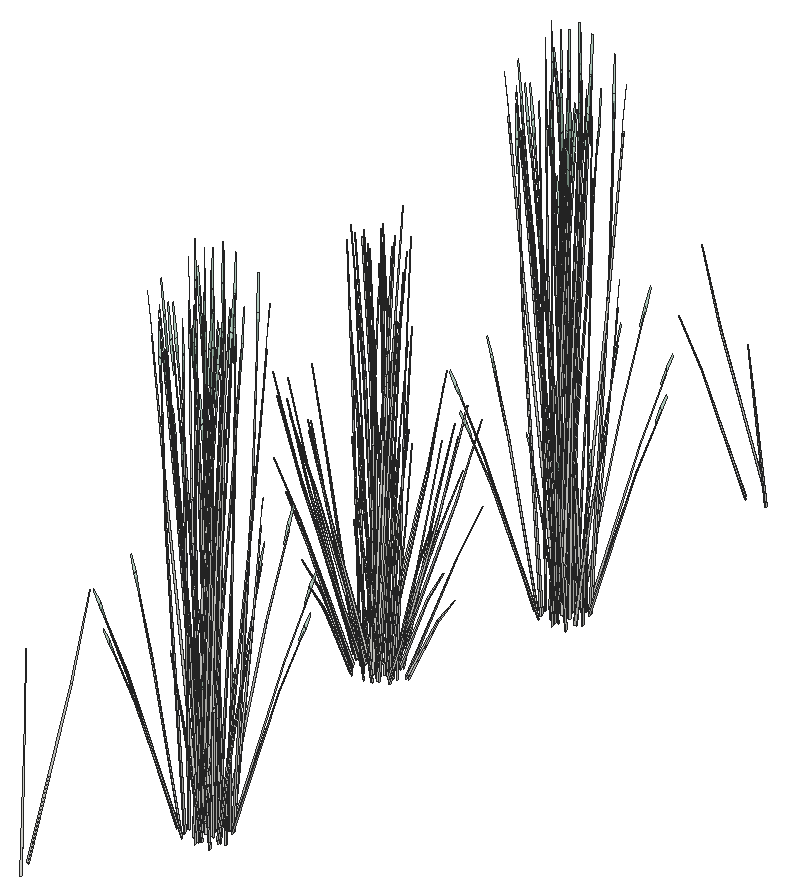
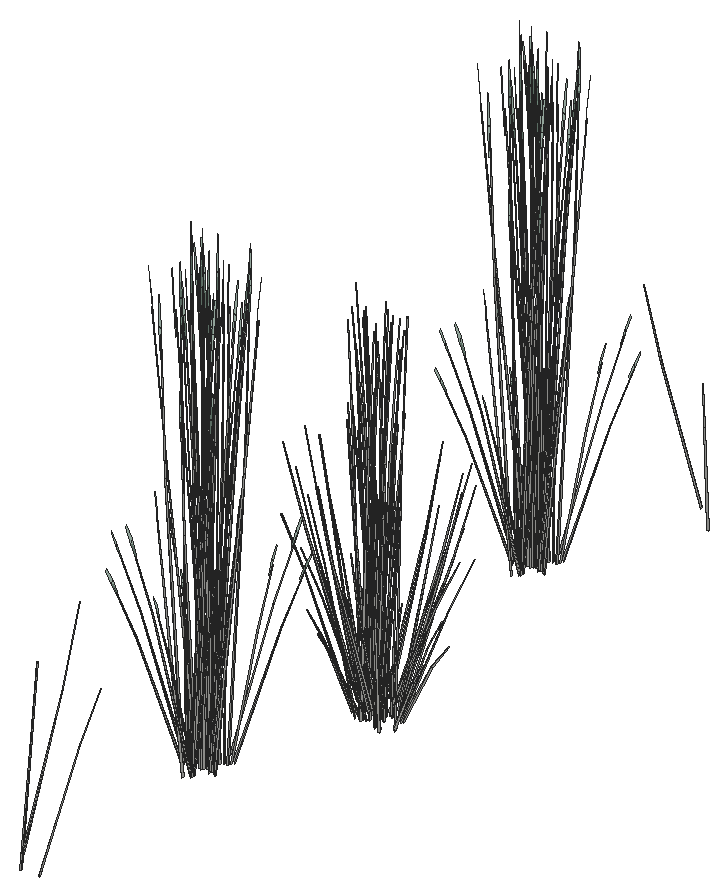
# SketchUp Ruby script. Lengths in inches.
U = 1.inch
M = Sketchup.active_model
def pt(a) = Geom::Point3d.new(a.map { |v| v * U })
def face(e, loops, mat)
  f = e.add_face(loops[0].map { |a| pt(a) })
  loops[1..].each { |l| e.add_face(l.map { |a| pt(a) }).erase! }
  f.material = f.back_material = mat if mat
  f
end
# faces: each face lists its corners as indices into pts; further lists are holes
def faces(e, pts, list, mat = nil) = list.each { |f| face(e, (f[0].is_a?(Array) ? f : [f]).map { |l| l.map { |i| pts[i] } }, mat) }
# xy, xz, yz: faces in a plane at the given z, y or x. An outline is a flat list of corners, or four numbers for a rectangle; further outlines are holes
def ring(l) = l.size == 4 ? [[l[0], l[1]], [l[2], l[1]], [l[2], l[3]], [l[0], l[3]]] : l.each_slice(2).to_a
def flat(e, list, mat, &to3) = list.each { |f| face(e, (f[0].is_a?(Array) ? f : [f]).map { |l| ring(l).map { |u, v| to3.(u, v) } }, mat) }
def xy(e, z, list, mat = nil) = flat(e, list, mat) { |x, y| [x, y, z] }
def xz(e, y, list, mat = nil) = flat(e, list, mat) { |x, z| [x, y, z] }
def yz(e, x, list, mat = nil) = flat(e, list, mat) { |y, z| [x, y, z] }
def lines(e, pts, list) = list.each { |a, b| e.add_line(pt(pts[a]), pt(pts[b])) }
# prism: a flat outline (further loops are holes) pulled along v
def prism(e, loops, v, mat = nil)
  f = face(e, loops, mat); d = Geom::Vector3d.new(v.map { |x| x * U })
  f.pushpull(f.normal.samedirection?(d) ? d.length : -d.length)
end
def box(e, o, s, mat = nil) = prism(e, [[o, [o[0] + s[0], o[1], o[2]], [o[0] + s[0], o[1] + s[1], o[2]], [o[0], o[1] + s[1], o[2]]]], [0, 0, s[2]], mat)
def at(x, y, z, deg = 0) = Geom::Transformation.translation(pt([x, y, z])) * Geom::Transformation.rotation(ORIGIN, Z_AXIS, deg.degrees)
def axes(o, x, y, z) = Geom::Transformation.new([*x, 0, *y, 0, *z, 0, *pt(o).to_a, 1])
def part(name) = M.definitions.add(name)
# library, detail: a bought-in or finely detailed component or shape, given as its bounding box
def library(name, o, s) = part(name).tap { |d| box(d.entities, o, s) }
def detail(e, o, s) = box(e.add_group.entities, o, s)
def put(e, d, t, mat = nil) = e.add_instance(d, t).tap { |i| i.material = mat if mat }
def group(e, t, mat = nil) = e.add_group.tap { |g| g.transformation = t; g.material = mat if mat }.entities
root = M.entities
M.materials.add("LightPink_Translucent").color = [175, 214, 192]
M.materials["LightPink_Translucent"].alpha = 0.75
c1 = part("blade")
p = [[2.15,0.21,22],[0,0.17,0],[0.09,0.45,0],[2.18,0.31,22],[2.29,0.31,22],[0.38,0.45,0],
  [2.48,0.24,33],[2.49,0.24,33],[2.48,0.22,33]]
faces(c1.entities,p,[[0,1,2,3],[4,5,2,3],[6,3,4,7],[8,0,3,6]])
c2 = part("blade with seeds\#1")
put(c2.entities,c1,at(0,0,0))
c3 = part("seeds")
p = [[0.3,-0.1,1.38],[-0.01,-0.03,1.59],[-0.01,-0.03,0.03],[0.14,-0.07,-0.07],[0.29,-0.03,3],[0.15,0.01,3.11]]
faces(c3.entities,p,[[0,1,2,3],[1,0,4,5]],"LightPink_Translucent")
c4 = part("blade with seeds")
put(c4.entities,c1,at(0,0,0))
put(c4.entities,c3,axes([2.4,0.25,30.99],[1.5799,-0.05474,1.17369],[-0.12525,1.92788,0.29478],[-0.07173,-0.02425,1.56792]))
put(root,c2,axes([485.82,259.22,140.8],[0.23727,0.30983,-0.58282],[-0.48842,0.17267,0.07033],[0.05548,0.1497,0.82446]))
put(root,c2,axes([484.45,259.71,138.84],[0.15688,-0.06011,1.17311],[0.38733,0.18125,-0.25229],[-0.11528,0.15683,0.50157]))
put(root,c4,axes([492.18,272.91,139.53],[-0.03656,0.1661,1.30132],[-0.37341,0.10705,-0.27986],[-0.0699,-0.22562,0.55638]))
put(root,c4,axes([493.98,273.55,139.53],[-0.12399,0.09331,1.30132],[-0.33702,-0.21502,-0.27986],[0.08055,-0.22079,0.55638]))
put(root,c4,axes([491.39,274.43,139.33],[-0.44625,-0.29882,0],[0.24886,-0.49993,-0.46963],[0.05668,-0.11386,1.48977]))
put(root,c4,axes([490.75,273.89,139.53],[0.07025,0.15082,1.30132],[-0.21183,0.37238,-0.27986],[-0.18329,-0.11083,0.55638]))
put(root,c4,axes([494.75,273.67,139.11],[-0.36364,-0.13787,-0.03542],[0.11186,-0.42434,-0.16061],[0.05948,-0.06443,0.52975]))
put(root,c4,axes([495.21,274.31,139.53],[-0.14568,-0.02894,1.30132],[-0.12195,-0.4231,-0.27986],[0.1883,-0.0989,0.55638]))
put(root,c4,axes([493.09,273.45,139.33],[0,-0.59763,0],[0.49772,0,-0.46963],[0.11336,0,1.48977]))
put(root,c4,axes([493.23,273.91,139.29],[-0.37441,-0.44456,0.27988],[0.37047,-0.44483,-0.33208],[0.10632,-0.01552,1.50045]))
put(root,c4,axes([492.3125,275.92,139.41],[0.35844,-0.4667,-0.22925],[0.40249,0.39271,0.50168],[-0.04193,-0.12567,1.53076]))
put(root,c4,axes([491.63,274.69,139.43],[-0.22267,0.44731,0.45182],[-0.39927,-0.26736,0],[0.05071,-0.10188,1.43328]))
put(root,c4,axes([492.44,275.11,139.39],[0.5277,0.12668,-0.2132],[-0.09198,0.60063,0.46656],[0.07287,-0.10495,1.42361]))
put(root,c4,axes([492.32,275.33,139.55],[-0.39744,-0.0922,0.13176],[0.06899,-0.45047,-0.37626],[0.04081,-0.08198,1.15337]))
put(root,c4,axes([493.02,273.81,139.43],[-0.44533,0,0.45182],[0,-0.53472,0],[0.10143,0,1.43328]))
put(root,c4,axes([491.33,276.26,139.17],[0.44781,-0.29509,-0.04679],[0.24886,0.49993,0.46963],[-0.04264,-0.12319,1.48904]))
put(root,c4,axes([491.09,273.99,139.74],[0.07886,0.43418,0.05922],[-0.31771,0.09982,-0.78537],[-0.16083,-0.02753,0.70398]))
put(root,c4,axes([495.22,275.32,139.11],[-0.25548,-0.33028,-0.03542],[0.27981,-0.30262,-0.16061],[0.07928,-0.02131,0.52975]))
put(root,c4,axes([492.7,275.18,139.32],[-0.09383,0.60408,0.41637],[-0.52992,-0.12294,0.16339],[0.05117,-0.08828,1.44559]))
put(root,c4,axes([491.85,274.86,139.42],[0.1182,0.51358,0.16054],[-0.43988,0.12682,0.31929],[0.06409,-0.0458,1.4597]))
put(root,c4,axes([491.78,275.52,139.17],[0.19993,-0.48183,0],[0.41543,0.23189,0],[0,0,1.48063]))
put(root,c4,axes([491.28,276.63,139.33],[-0.44625,0.29882,0],[-0.24886,-0.49993,-0.46963],[-0.05668,-0.11386,1.48977]))
put(root,c4,axes([491.83,276.39,139.42],[0.44258,0.13807,0.16054],[-0.12525,0.50524,0.31929],[-0.00216,-0.08728,1.4597]))
put(root,c4,axes([492.42,276.15,139.55],[-0.26757,0.3531,0.13176],[-0.30187,-0.29453,-0.37626],[-0.04081,-0.08198,1.15337]))
put(root,c4,axes([492.75,276.03,139.26],[0.3833,-0.44456,-0.05579],[0.38354,0.44483,0],[0.01339,-0.01552,1.5977]))
put(root,c4,axes([491.5625,276.27,139.29],[-0.14475,0.59835,0.27988],[-0.51739,-0.14969,-0.33208],[-0.06475,-0.09903,1.50045]))
put(root,c4,axes([491.59,276.53,139.43],[0.22267,0.44731,0.45182],[-0.39927,0.26736,0],[-0.05071,-0.10188,1.43328]))
put(root,c4,axes([493.1875,275.13,139.32],[-0.49797,0.2078,0.41637],[-0.17316,-0.59373,0.16339],[0.0915,0.00726,1.44559]))
put(root,c4,axes([491.96,275.63,139.18],[0.38394,-0.15594,0],[0.13445,0.4453,0],[0,0,1.40478]))
put(root,c4,axes([492.96,277.18,139.42],[0.32439,-0.37551,0.16054],[0.31463,0.37842,0.31929],[-0.06625,-0.04147,1.4597]))
put(root,c4,axes([493.14,275.88,139.18],[0.51528,0,0],[0,0.59763,0],[0,0,1.63305]))
put(root,c4,axes([493.05,275.32,139.38],[-0.21584,0.53851,0.21899],[-0.44849,-0.25917,0.45502],[0.10338,0,1.46094]))
put(root,c4,axes([492.9375,276.18,139.26],[-0.51503,0,-0.0513],[0,-0.59763,0],[-0.01619,0,1.63225]))
put(root,c4,axes([494.13,274.91,139.42],[-0.44258,-0.13807,0.16054],[0.12525,-0.50524,0.31929],[0.00216,0.08728,1.4597]))
put(root,c4,axes([491.94,275.89,139.25],[-0.51161,0.2078,-0.05471],[-0.17927,-0.59373,0],[-0.01787,0.00726,1.56677]))
put(root,c4,axes([494.68,274.66,139.33],[0.44625,-0.29882,0],[0.24886,0.49993,-0.46963],[0.05668,0.11386,1.48977]))
put(root,c4,axes([492.61,277.61,139.17],[0.00356,-0.59734,-0.04529],[0.49772,0,0.45448],[-0.1133,-0.01877,1.441]))
put(root,c4,axes([494.11,276.4375,139.42],[-0.1182,-0.51358,0.16054],[0.43988,-0.12682,0.31929],[-0.06409,0.0458,1.4597]))
put(root,c4,axes([493.47,275.6,139.32],[-0.40415,-0.39628,0.41637],[0.35675,-0.4708,0.16339],[0.04033,0.09554,1.44559]))
put(root,c4,axes([492.83,276.27,139.19],[-0.28765,0.33362,0],[-0.28765,-0.33362,0],[0,0,1.54032]))
put(root,c4,axes([491.77,276.07,139.18],[-0.19993,0.48183,0],[-0.41543,-0.23189,0],[0,0,1.59208]))
put(root,c4,axes([493.26,276.11,139.34],[0.09383,-0.60408,0.44771],[0.52992,0.12294,0.17569],[-0.05117,0.08828,1.5544]))
put(root,c4,axes([493.03,276.28,139.18],[0,0.53472,0],[-0.46104,0,0],[0,0,1.6235]))
put(root,c4,axes([493.08,276.47,139.55],[0.12987,0.4453,0.13176],[-0.37086,0.15594,-0.37626],[-0.08162,0,1.15337]))
put(root,c4,axes([495.04,276.41,139.53],[-0.09014,-0.13585,1.30132],[0.15777,-0.40687,-0.27986],[0.19621,0.07542,0.55638]))
put(root,c4,axes([492.94,277.49,139.43],[0.44533,0,0.45182],[0,0.53472,0],[-0.10143,0,1.43328]))
put(root,c4,axes([493.64,275.96,139.55],[0.39744,0.0922,0.13176],[-0.06899,0.45047,-0.37626],[-0.04081,0.08198,1.15337]))
put(root,c4,axes([494.34,276.6,139.43],[0.22267,-0.44731,0.45182],[0.39927,0.26736,0],[-0.05071,0.10188,1.43328]))
put(root,c4,axes([492.01,276.21,139.16],[0.1511,0.50177,-0.1747],[-0.43526,0.17632,0.00007],[0.0167,0.05539,1.58246]))
put(root,c4,axes([491.74,276.08,139.53],[0.14762,0.00843,1.30132],[0.1649,0.40305,-0.27986],[-0.17669,0.12442,0.55638]))
put(root,c4,axes([492.87,277.85,139.33],[0,0.59763,0],[-0.49772,0,-0.46963],[-0.11336,0,1.48977]))
put(root,c4,axes([494.57,276.86,139.33],[0.44625,0.29882,0],[-0.24886,0.49993,-0.46963],[-0.05668,0.11386,1.48977]))
put(root,c4,axes([493.18,278.6,139.23],[0.28477,-0.29631,-0.05904],[0.26092,0.32453,-0.26768],[0.01837,0.09195,0.88292]))
put(root,c4,axes([493.98,277.72,139.53],[0.01319,-0.17074,1.30132],[0.35385,-0.17492,-0.27986],[0.1001,0.20976,0.55638]))
put(root,c4,axes([492.8,278.04,138.97],[-0.05344,-0.30783,1.28841],[0.4254,-0.049,0.07375],[0.06439,0.2156,0.73315]))
put(root,c4,axes([492.17,278.125,139.53],[0.10953,-0.1151,1.30132],[0.36232,0.14976,-0.27986],[-0.04908,0.23288,0.55638]))
put(root,c2,axes([487.07,306.03,138.84],[-0.14131,0.07713,1.17311],[-0.4232,-0.13499,-0.25229],[0.07845,-0.16789,0.50157]))
put(root,c2,axes([486.43,306.29,140.8],[-0.23727,-0.30983,-0.58282],[0.48842,-0.17267,0.07033],[-0.05548,-0.1497,0.82446]))
put(root,c2,axes([484.89,305.88,138.84],[-0.0301,0.12465,1.17311],[-0.44009,0.10435,-0.25229],[-0.10287,-0.16111,0.50157]))
put(root,c2,axes([487.42,306.6,140.8],[0.01294,-0.35246,-0.58282],[0.54471,0.02367,0.07033],[0.05748,-0.14932,0.82446]))
put(root,c2,axes([486.55,305.41,138.99],[0.06377,0.2222,0.94226],[-0.35378,-0.12306,0.69231],[0.03807,-0.11377,0.20754]))
put(root,c2,axes([486.25,306.23,140.56],[-0.48869,-0.09552,-0.41919],[0.16751,-0.3275,-0.3247],[-0.04481,-0.13186,0.80208]))
put(root,c2,axes([487.31,306.48,140.56],[-0.35588,-0.25603,-0.41919],[0.37594,-0.22422,-0.3247],[0.05415,-0.13008,0.80208]))
put(root,c2,axes([484.73,305.68,138.99],[0.25932,0.13262,0.94226],[-0.37767,0.07972,0.69231],[-0.08081,-0.10192,0.20754]))
put(root,c2,axes([485.36,306.38,140.8],[-0.4239,-0.18418,-0.58282],[0.30126,-0.32274,0.07033],[-0.15358,-0.10997,0.82446]))
put(root,c2,axes([485.16,306.39,140.56],[-0.49056,0.09058,-0.41919],[-0.08581,-0.34303,-0.3247],[-0.13176,-0.0983,0.80208]))
put(root,c2,axes([488.05,307.07,140.56],[-0.12771,-0.34793,-0.41919],[0.48364,-0.06086,-0.3247],[0.1386,-0.09345,0.80208]))
put(root,c2,axes([488.06,307.21,140.8],[0.25968,-0.30066,-0.58282],[0.45504,0.21367,0.07033],[0.15505,-0.10893,0.82446]))
put(root,c2,axes([488.43,306.93,138.84],[-0.1776,-0.01129,1.17311],[-0.18194,-0.30276,-0.25229],[0.21818,-0.08565,0.50157]))
put(root,c2,axes([488.64,306.375,138.99],[-0.16559,0.19397,0.94226],[-0.14233,-0.26061,0.69231],[0.13676,-0.0653,0.20754]))
put(root,c2,axes([484.09,306.93,138.84],[0.09706,0.10609,1.17311],[-0.22366,0.28837,-0.25229],[-0.22965,-0.06892,0.50157]))
put(root,c2,axes([484.5,306.84,140.8],[-0.49695,-0.00917,-0.58282],[0.03338,-0.38634,0.07033],[-0.21053,-0.04077,0.82446]))
put(root,c2,axes([484.33,306.92,140.56],[-0.36098,0.25241,-0.41919],[-0.31614,-0.26664,-0.3247],[-0.18341,-0.0384,0.80208]))
put(root,c2,axes([485.94,307.73,138.71],[0.56014,0.18468,0.19741],[-0.26958,0.38374,0.41019],[0,-0.08846,1.31701]))
put(root,c2,axes([483.52,307.25,138.99],[0.31739,-0.02727,0.94226],[-0.20133,0.24024,0.69231],[-0.15684,-0.03604,0.20754]))
put(root,c2,axes([485.76,307.47,138.95],[-0.53984,0.02352,0.36702],[-0.04882,-0.39046,-0.17663],[0.09664,-0.03957,1.17838]))
put(root,c2,axes([484.37,307.76,138.75],[0,0.38104,0.40731],[-0.5562,0,0],[0,-0.08679,1.29208]))
put(root,c2,axes([485.74,307.61,138.65],[0.21614,0.42608,0.37535],[-0.61757,0.14817,0.14729],[0.00755,-0.07829,1.30318]))
put(root,c2,axes([488.27,307.84,140.56],[0.13468,-0.34661,-0.41919],[0.46175,0.1188,-0.3247],[0.18591,-0.03178,0.80208]))
put(root,c2,axes([487.27,306.63,138.75],[-0.46527,-0.19052,0.40731],[0.2781,-0.34163,0],[0.10597,0.04339,1.29208]))
put(root,c2,axes([485.63,307.95,138.95],[-0.2412,0.34335,0.36702],[-0.50118,-0.16524,-0.17663],[0,-0.07915,1.17838]))
put(root,c2,axes([486.22,307.37,138.65],[-0.41219,0.3458,0.37535],[-0.4897,-0.30525,0.14729],[0.09937,-0.03451,1.30318]))
put(root,c2,axes([485.51,306.8,138.75],[-0.14361,0.37869,0.14473],[-0.52552,-0.10717,0.28783],[0.09078,-0.00184,1.3159]))
put(root,c2,axes([488.18,307.97,140.8],[0.43684,-0.16829,-0.58282],[0.24345,0.34641,0.07033],[0.21107,-0.03935,0.82446]))
put(root,c2,axes([486.61,307.22,138.86],[0.0959,-0.34006,0.11878],[0.46856,0.05903,-0.33919],[0.08527,0.03492,1.03975]))
put(root,c2,axes([486.41,307.3125,138.95],[-0.29864,-0.31983,0.36702],[0.45236,-0.22522,-0.17663],[0.09664,0.03957,1.17838]))
put(root,c2,axes([485.8,308.03,138.65],[0.62833,0.08028,0.37535],[-0.12787,0.45342,0.14729],[-0.09182,-0.04378,1.30318]))
put(root,c2,axes([487.1,306.82,138.75],[-0.5342,0.10113,0.14473],[-0.13191,-0.37638,0.28783],[0.04764,0.05484,1.3159]))
put(root,c2,axes([485.46,308.75,138.75],[0.5342,-0.10113,0.14473],[0.13191,0.37638,0.28783],[-0.04764,-0.05484,1.3159]))
put(root,c2,axes([486.76,307.55,138.67],[-0.62833,-0.08028,0.4036],[0.12787,-0.45342,0.15838],[0.09182,0.04378,1.40127]))
put(root,c2,axes([485.95,308.35,138.86],[-0.0959,0.34006,0.11878],[-0.46856,-0.05903,-0.33919],[-0.08527,-0.03492,1.03975]))
put(root,c2,axes([487.87,307.81,138.75],[-0.39059,-0.27756,0.14473],[0.39362,-0.26921,0.28783],[-0.04314,0.05668,1.3159]))
put(root,c2,axes([484.96,307.45,139.46],[0.14131,-0.05512,1.45254],[0.04873,0.38487,0.11368],[-0.30608,0.05107,0.51915]))
put(root,c2,axes([489.43,308.0625,138.99],[-0.30716,0.06291,0.94226],[0.14458,-0.25998,0.69231],[0.16295,0.01779,0.20754]))
put(root,c2,axes([487.05,308.78,138.75],[0.14361,-0.37869,0.14473],[0.52552,0.10717,0.28783],[-0.09078,0.00184,1.3159]))
put(root,c2,axes([486.92,307.63,138.95],[0.2412,-0.34335,0.36702],[0.50118,0.16524,-0.17663],[0,0.07915,1.17838]))
put(root,c2,axes([485.28,308.95,138.75],[0.46527,0.19052,0.40731],[-0.2781,0.34163,0],[-0.10597,-0.04339,1.29208]))
put(root,c2,axes([483.98,307.66,140.56],[-0.13468,0.34661,-0.41919],[-0.46175,-0.1188,-0.3247],[-0.18591,0.03178,0.80208]))
put(root,c2,axes([488.1875,307.82,138.75],[0,-0.38104,0.40731],[0.5562,0,0],[0,0.08679,1.29208]))
put(root,c2,axes([487.13,307.71,138.86],[0.46318,-0.11112,0.11878],[0.1622,0.31732,-0.33919],[0,0.06984,1.03975]))
put(root,c2,axes([486.8,308.1,138.95],[0.53984,-0.02352,0.36702],[0.04882,0.39046,-0.17663],[-0.09664,0.03957,1.17838]))
put(root,c2,axes([488.85,308.48,138.84],[-0.11973,-0.09372,1.17311],[0.15578,-0.31002,-0.25229],[0.24224,0.042,0.50157]))
put(root,c2,axes([486.8,308.27,138.86],[0.36728,0.22894,0.11878],[-0.30636,0.25829,-0.33919],[-0.08527,0.03492,1.03975]))
put(root,c2,axes([487.76,308.67,140.8],[0.49695,0.00917,-0.58282],[-0.03338,0.38634,0.07033],[0.21053,0.04077,0.82446]))
put(root,c2,axes([487.2,308.98,138.75],[0.46527,-0.19052,0.40731],[0.2781,0.34163,0],[-0.10597,0.04339,1.29208]))
put(root,c2,axes([483.43,308.48,138.84],[0.17277,0.03128,1.17311],[0.11135,0.3195,-0.25229],[-0.23468,0.05981,0.50157]))
put(root,c2,axes([483.07,309.15,138.99],[0.20718,-0.1727,0.94226],[0.08175,0.27339,0.69231],[-0.14972,0.04895,0.20754]))
put(root,c2,axes([487.72,308.96,138.99],[-0.27991,-0.10956,0.94226],[0.36143,-0.11132,0.69231],[0.09749,0.0943,0.20754]))
put(root,c2,axes([484.21,308.4375,140.56],[0.12771,0.34793,-0.41919],[-0.48364,0.06086,-0.3247],[-0.1386,0.09345,0.80208]))
put(root,c2,axes([487.04,307.73,139.05],[-0.01358,-0.35877,1.15892],[0.61462,0.093,0.4907],[-0.14537,0.19631,1.09393]))
put(root,c2,axes([487.09,309.11,140.56],[0.49056,-0.09058,-0.41919],[0.08581,0.34303,-0.3247],[0.13176,0.0983,0.80208]))
put(root,c2,axes([487.77,309.46,138.91],[-0.31879,-0.01195,0.86186],[0.21053,-0.25381,0.47585],[0.12594,0.09017,0.67605]))
put(root,c2,axes([486.73,308.85,138.84],[0.00877,-0.12631,1.17311],[0.41923,-0.14109,-0.25229],[0.12942,0.15118,0.50157]))
put(root,c2,axes([484.82,309.9,138.99],[-0.01287,-0.22657,0.94226],[0.32149,0.1616,0.69231],[-0.06323,0.10799,0.20754]))
put(root,c2,axes([486,309.27,140.56],[0.48869,0.09552,-0.41919],[-0.16751,0.3275,-0.3247],[0.04481,0.13186,0.80208]))
put(root,c2,axes([484.56,309.41,139.03],[0.45162,-0.06748,0.05338],[0.10383,0.27185,-0.708],[-0.02863,0.13761,0.63462]))
put(root,c2,axes([484.83,308.91,141.1],[-0.01294,0.35246,-0.64693],[-0.54471,-0.02367,0.07807],[-0.05748,0.14932,0.91515]))
put(root,c2,axes([485.82,309.21,140.8],[0.23727,0.30983,-0.58282],[-0.48842,0.17267,0.07033],[0.05548,0.1497,0.82446]))
put(root,c2,axes([484.45,309.7,138.84],[0.15688,-0.06011,1.17311],[0.38733,0.18125,-0.25229],[-0.11528,0.15683,0.50157]))
put(root,c4,axes([492.18,322.89,139.53],[-0.03656,0.1661,1.30132],[-0.37341,0.10705,-0.27986],[-0.0699,-0.22562,0.55638]))
put(root,c4,axes([493.98,323.54,139.53],[-0.12399,0.09331,1.30132],[-0.33702,-0.21502,-0.27986],[0.08055,-0.22079,0.55638]))
put(root,c4,axes([491.39,324.42,139.33],[-0.44625,-0.29882,0],[0.24886,-0.49993,-0.46963],[0.05668,-0.11386,1.48977]))
put(root,c4,axes([490.75,323.875,139.53],[0.07025,0.15082,1.30132],[-0.21183,0.37238,-0.27986],[-0.18329,-0.11083,0.55638]))
put(root,c4,axes([494.75,323.66,139.11],[-0.36364,-0.13787,-0.03542],[0.11186,-0.42434,-0.16061],[0.05948,-0.06443,0.52975]))
put(root,c4,axes([495.21,324.3,139.53],[-0.14568,-0.02894,1.30132],[-0.12195,-0.4231,-0.27986],[0.1883,-0.0989,0.55638]))
put(root,c4,axes([493.09,323.43,139.33],[0,-0.59763,0],[0.49772,0,-0.46963],[0.11336,0,1.48977]))
put(root,c4,axes([493.23,323.9,139.29],[-0.37441,-0.44456,0.27988],[0.37047,-0.44483,-0.33208],[0.10632,-0.01552,1.50045]))
put(root,c4,axes([492.3125,325.91,139.41],[0.35844,-0.4667,-0.22925],[0.40249,0.39271,0.50168],[-0.04193,-0.12567,1.53076]))
put(root,c4,axes([491.63,324.68,139.43],[-0.22267,0.44731,0.45182],[-0.39927,-0.26736,0],[0.05071,-0.10188,1.43328]))
put(root,c4,axes([492.44,325.1,139.39],[0.5277,0.12668,-0.2132],[-0.09198,0.60063,0.46656],[0.07287,-0.10495,1.42361]))
put(root,c4,axes([492.32,325.32,139.55],[-0.39744,-0.0922,0.13176],[0.06899,-0.45047,-0.37626],[0.04081,-0.08198,1.15337]))
put(root,c4,axes([493.02,323.8,139.43],[-0.44533,0,0.45182],[0,-0.53472,0],[0.10143,0,1.43328]))
put(root,c4,axes([491.33,326.25,139.17],[0.44781,-0.29509,-0.04679],[0.24886,0.49993,0.46963],[-0.04264,-0.12319,1.48904]))
put(root,c4,axes([491.09,323.98,139.74],[0.07886,0.43418,0.05922],[-0.31771,0.09982,-0.78537],[-0.16083,-0.02753,0.70398]))
put(root,c4,axes([495.22,325.3,139.11],[-0.25548,-0.33028,-0.03542],[0.27981,-0.30262,-0.16061],[0.07928,-0.02131,0.52975]))
put(root,c4,axes([492.7,325.17,139.32],[-0.09383,0.60408,0.41637],[-0.52992,-0.12294,0.16339],[0.05117,-0.08828,1.44559]))
put(root,c4,axes([491.85,324.85,139.42],[0.1182,0.51358,0.16054],[-0.43988,0.12682,0.31929],[0.06409,-0.0458,1.4597]))
put(root,c4,axes([491.78,325.51,139.17],[0.19993,-0.48183,0],[0.41543,0.23189,0],[0,0,1.48063]))
put(root,c4,axes([491.28,326.62,139.33],[-0.44625,0.29882,0],[-0.24886,-0.49993,-0.46963],[-0.05668,-0.11386,1.48977]))
put(root,c4,axes([491.83,326.375,139.42],[0.44258,0.13807,0.16054],[-0.12525,0.50524,0.31929],[-0.00216,-0.08728,1.4597]))
put(root,c4,axes([492.42,326.14,139.55],[-0.26757,0.3531,0.13176],[-0.30187,-0.29453,-0.37626],[-0.04081,-0.08198,1.15337]))
put(root,c4,axes([492.75,326.02,139.26],[0.3833,-0.44456,-0.05579],[0.38354,0.44483,0],[0.01339,-0.01552,1.5977]))
put(root,c4,axes([491.5625,326.26,139.29],[-0.14475,0.59835,0.27988],[-0.51739,-0.14969,-0.33208],[-0.06475,-0.09903,1.50045]))
put(root,c4,axes([491.59,326.52,139.43],[0.22267,0.44731,0.45182],[-0.39927,0.26736,0],[-0.05071,-0.10188,1.43328]))
put(root,c4,axes([493.1875,325.12,139.32],[-0.49797,0.2078,0.41637],[-0.17316,-0.59373,0.16339],[0.0915,0.00726,1.44559]))
put(root,c4,axes([491.96,325.62,139.18],[0.38394,-0.15594,0],[0.13445,0.4453,0],[0,0,1.40478]))
put(root,c4,axes([492.96,327.16,139.42],[0.32439,-0.37551,0.16054],[0.31463,0.37842,0.31929],[-0.06625,-0.04147,1.4597]))
put(root,c4,axes([493.14,325.87,139.18],[0.51528,0,0],[0,0.59763,0],[0,0,1.63305]))
put(root,c4,axes([493.05,325.3125,139.38],[-0.21584,0.53851,0.21899],[-0.44849,-0.25917,0.45502],[0.10338,0,1.46094]))
put(root,c4,axes([492.9375,326.17,139.26],[-0.51503,0,-0.0513],[0,-0.59763,0],[-0.01619,0,1.63225]))
put(root,c4,axes([494.13,324.9,139.42],[-0.44258,-0.13807,0.16054],[0.12525,-0.50524,0.31929],[0.00216,0.08728,1.4597]))
put(root,c4,axes([491.94,325.88,139.25],[-0.51161,0.2078,-0.05471],[-0.17927,-0.59373,0],[-0.01787,0.00726,1.56677]))
put(root,c4,axes([494.68,324.65,139.33],[0.44625,-0.29882,0],[0.24886,0.49993,-0.46963],[0.05668,0.11386,1.48977]))
put(root,c4,axes([492.61,327.6,139.17],[0.00356,-0.59734,-0.04529],[0.49772,0,0.45448],[-0.1133,-0.01877,1.441]))
put(root,c4,axes([494.11,326.42,139.42],[-0.1182,-0.51358,0.16054],[0.43988,-0.12682,0.31929],[-0.06409,0.0458,1.4597]))
put(root,c4,axes([493.47,325.58,139.32],[-0.40415,-0.39628,0.41637],[0.35675,-0.4708,0.16339],[0.04033,0.09554,1.44559]))
put(root,c4,axes([492.83,326.26,139.19],[-0.28765,0.33362,0],[-0.28765,-0.33362,0],[0,0,1.54032]))
put(root,c4,axes([491.77,326.05,139.18],[-0.19993,0.48183,0],[-0.41543,-0.23189,0],[0,0,1.59208]))
put(root,c4,axes([493.26,326.1,139.34],[0.09383,-0.60408,0.44771],[0.52992,0.12294,0.17569],[-0.05117,0.08828,1.5544]))
put(root,c4,axes([493.03,326.27,139.18],[0,0.53472,0],[-0.46104,0,0],[0,0,1.6235]))
put(root,c4,axes([493.08,326.46,139.55],[0.12987,0.4453,0.13176],[-0.37086,0.15594,-0.37626],[-0.08162,0,1.15337]))
put(root,c4,axes([495.04,326.4,139.53],[-0.09014,-0.13585,1.30132],[0.15777,-0.40687,-0.27986],[0.19621,0.07542,0.55638]))
put(root,c4,axes([492.94,327.47,139.43],[0.44533,0,0.45182],[0,0.53472,0],[-0.10143,0,1.43328]))
put(root,c4,axes([493.64,325.95,139.55],[0.39744,0.0922,0.13176],[-0.06899,0.45047,-0.37626],[-0.04081,0.08198,1.15337]))
put(root,c4,axes([494.34,326.59,139.43],[0.22267,-0.44731,0.45182],[0.39927,0.26736,0],[-0.05071,0.10188,1.43328]))
put(root,c4,axes([492.01,326.2,139.16],[0.1511,0.50177,-0.1747],[-0.43526,0.17632,0.00007],[0.0167,0.05539,1.58246]))
put(root,c4,axes([491.74,326.07,139.53],[0.14762,0.00843,1.30132],[0.1649,0.40305,-0.27986],[-0.17669,0.12442,0.55638]))
put(root,c4,axes([492.87,327.84,139.33],[0,0.59763,0],[-0.49772,0,-0.46963],[-0.11336,0,1.48977]))
put(root,c4,axes([494.57,326.85,139.33],[0.44625,0.29882,0],[-0.24886,0.49993,-0.46963],[-0.05668,0.11386,1.48977]))
put(root,c4,axes([493.18,328.59,139.23],[0.28477,-0.29631,-0.05904],[0.26092,0.32453,-0.26768],[0.01837,0.09195,0.88292]))
put(root,c4,axes([493.98,327.71,139.53],[0.01319,-0.17074,1.30132],[0.35385,-0.17492,-0.27986],[0.1001,0.20976,0.55638]))
put(root,c4,axes([492.8,328.02,138.97],[-0.05344,-0.30783,1.28841],[0.4254,-0.049,0.07375],[0.06439,0.2156,0.73315]))
put(root,c4,axes([492.17,328.11,139.53],[0.10953,-0.1151,1.30132],[0.36232,0.14976,-0.27986],[-0.04908,0.23288,0.55638]))
put(root,c2,axes([494.52,351.93,138.9375],[-0.14131,0.07713,1.17311],[-0.4232,-0.13499,-0.25229],[0.07845,-0.16789,0.50157]))
put(root,c2,axes([493.87,352.2,140.9],[-0.23727,-0.30983,-0.58282],[0.48842,-0.17267,0.07033],[-0.05548,-0.1497,0.82446]))
put(root,c2,axes([492.33,351.79,138.9375],[-0.0301,0.12465,1.17311],[-0.44009,0.10435,-0.25229],[-0.10287,-0.16111,0.50157]))
